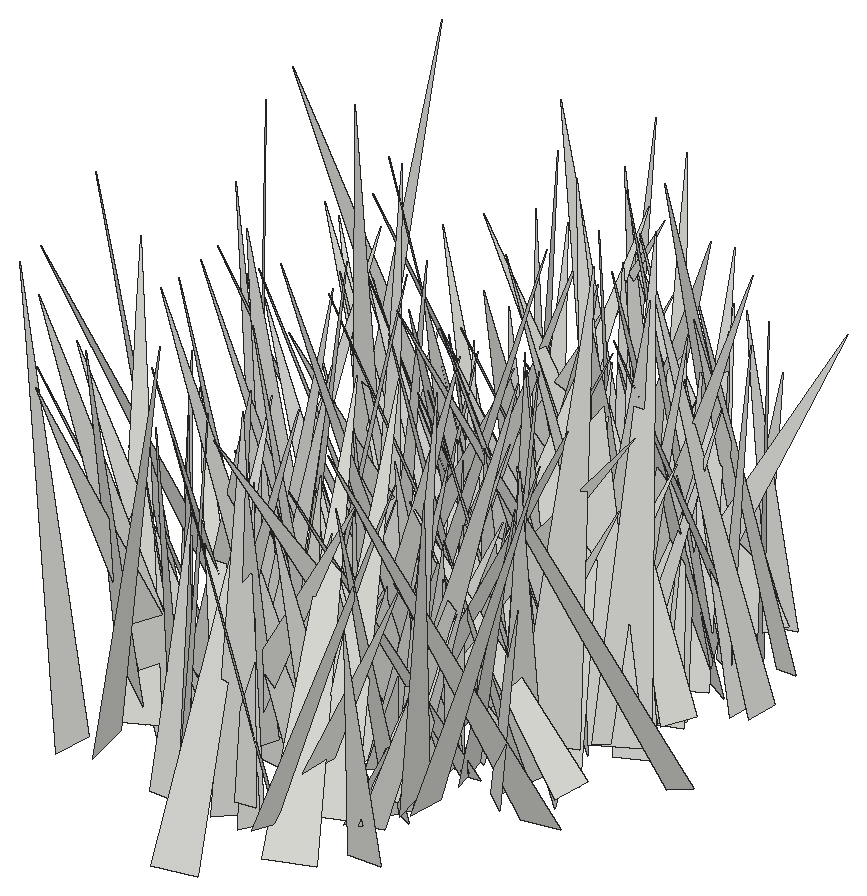
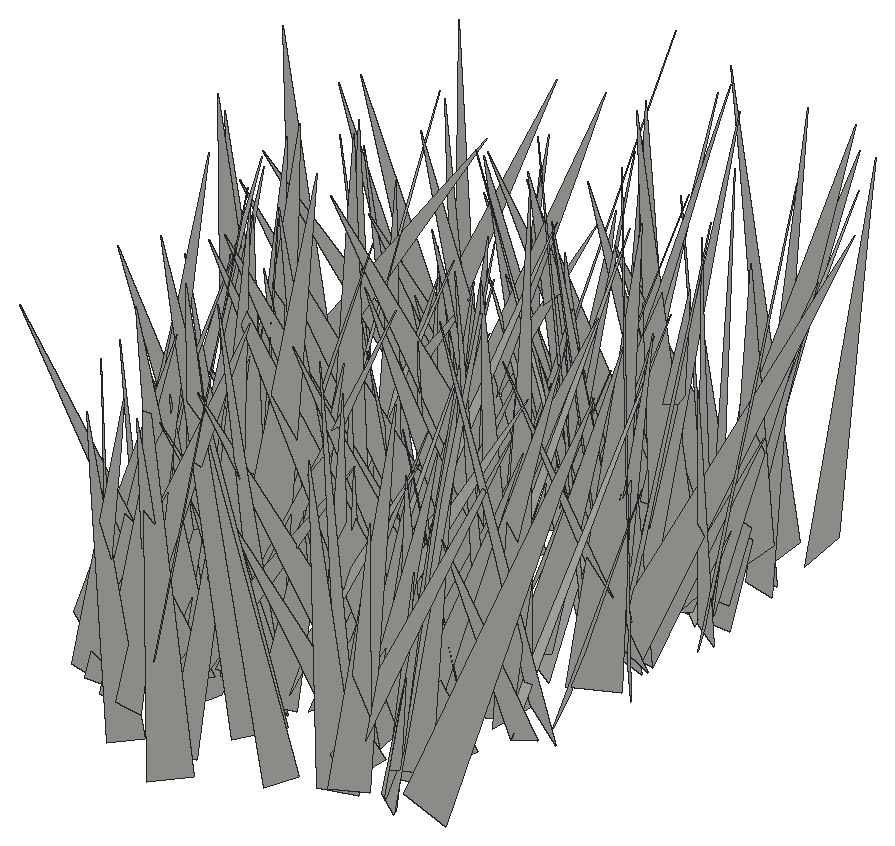
# SketchUp Ruby script. Lengths in inches.
U = 1.inch
M = Sketchup.active_model
def pt(a) = Geom::Point3d.new(a.map { |v| v * U })
def face(e, loops, mat)
  f = e.add_face(loops[0].map { |a| pt(a) })
  loops[1..].each { |l| e.add_face(l.map { |a| pt(a) }).erase! }
  f.material = f.back_material = mat if mat
  f
end
# faces: each face lists its corners as indices into pts; further lists are holes
def faces(e, pts, list, mat = nil) = list.each { |f| face(e, (f[0].is_a?(Array) ? f : [f]).map { |l| l.map { |i| pts[i] } }, mat) }
# xy, xz, yz: faces in a plane at the given z, y or x. An outline is a flat list of corners, or four numbers for a rectangle; further outlines are holes
def ring(l) = l.size == 4 ? [[l[0], l[1]], [l[2], l[1]], [l[2], l[3]], [l[0], l[3]]] : l.each_slice(2).to_a
def flat(e, list, mat, &to3) = list.each { |f| face(e, (f[0].is_a?(Array) ? f : [f]).map { |l| ring(l).map { |u, v| to3.(u, v) } }, mat) }
def xy(e, z, list, mat = nil) = flat(e, list, mat) { |x, y| [x, y, z] }
def xz(e, y, list, mat = nil) = flat(e, list, mat) { |x, z| [x, y, z] }
def yz(e, x, list, mat = nil) = flat(e, list, mat) { |y, z| [x, y, z] }
def lines(e, pts, list) = list.each { |a, b| e.add_line(pt(pts[a]), pt(pts[b])) }
# prism: a flat outline (further loops are holes) pulled along v
def prism(e, loops, v, mat = nil)
  f = face(e, loops, mat); d = Geom::Vector3d.new(v.map { |x| x * U })
  f.pushpull(f.normal.samedirection?(d) ? d.length : -d.length)
end
def box(e, o, s, mat = nil) = prism(e, [[o, [o[0] + s[0], o[1], o[2]], [o[0] + s[0], o[1] + s[1], o[2]], [o[0], o[1] + s[1], o[2]]]], [0, 0, s[2]], mat)
def at(x, y, z, deg = 0) = Geom::Transformation.translation(pt([x, y, z])) * Geom::Transformation.rotation(ORIGIN, Z_AXIS, deg.degrees)
def axes(o, x, y, z) = Geom::Transformation.new([*x, 0, *y, 0, *z, 0, *pt(o).to_a, 1])
def part(name) = M.definitions.add(name)
# library, detail: a bought-in or finely detailed component or shape, given as its bounding box
def library(name, o, s) = part(name).tap { |d| box(d.entities, o, s) }
def detail(e, o, s) = box(e.add_group.entities, o, s)
def put(e, d, t, mat = nil) = e.add_instance(d, t).tap { |i| i.material = mat if mat }
def group(e, t, mat = nil) = e.add_group.tap { |g| g.transformation = t; g.material = mat if mat }.entities
root = M.entities
c1 = part("fur_instance\#9")
p = [[0.8125,0,1.79],[0.67,-0.02,1.48],[0,-0.11,0],[0,0.11,0]]
faces(c1.entities,p,[[0,1,2,3]])
put(root,c1,axes([64.6,109.23,-27.1],[-0.79345,-6.87819,1.77521],[-6.83318,0.25089,-2.08208],[-1.94125,1.92821,6.60333]))
put(root,c1,axes([64.78,96.99,-27.1],[-6.58446,-3.61184,1.85584],[-3.84727,6.67992,-0.64953],[1.29924,1.4758,7.48189]))
put(root,c1,axes([66.12,98.6,-27.1],[-2.71774,-6.73125,0.47193],[-6.54696,2.5072,-1.9416],[-1.63394,1.15011,6.99472]))
put(root,c1,axes([65.09,91.46,-27.1],[-7.05246,-0.20222,1.59365],[-0.38202,7.18084,-0.77939],[1.56034,0.84409,7.01218]))
put(root,c1,axes([66.34,101.17,-28.22],[-5.41168,-1.42657,0.35166],[-1.45652,5.03228,-1.99993],[-0.1932,2.0214,5.22701]))
put(root,c1,axes([64.6875,96.98,-27.1],[1.72426,4.07776,1.35625],[4.04188,-2.03524,0.98061],[-1.4597,-0.81871,4.31736]))
put(root,c1,axes([65.79,93.5625,-27.1],[-1.06159,6.87885,0.56166],[6.76624,0.92524,1.45707],[-1.36093,-0.76575,6.80607]))
put(root,c1,axes([65.8,96.19,-27.1],[-4.26864,3.3889,1.68719],[3.78174,3.93314,1.66776],[0.17248,-2.36607,5.18889]))
put(root,c1,axes([66.37,104.19,-27.1],[-3.43494,4.07646,0.13435],[4.04677,3.38429,0.77755],[-0.50915,-0.60283,5.27368]))
put(root,c1,axes([64.64,100.35,-27.1],[-5.7343,-4.84539,3.53032],[-5.45543,6.24306,-0.29262],[2.4858,2.5238,7.50162]))
put(root,c1,axes([65.6,104.33,-27.1],[-4.61159,-4.4726,0.38091],[-4.39573,4.61032,0.9157],[0.90928,-0.396,6.35865]))
put(root,c1,axes([65.06,103.58,-27.1],[3.59561,7.30217,1.1805],[7.09033,-3.77639,1.76345],[-2.10771,-0.24675,7.94609]))
put(root,c1,axes([65.57,96.5,-27.1],[-4.43936,-4.76816,0.23664],[-4.66276,4.39992,1.18262],[1.02469,-0.63608,6.40661]))
put(root,c1,axes([66.47,97.26,-28.22],[-2.53868,-3.44184,0.53172],[-3.38696,2.28677,-1.36858],[-0.81085,1.22404,4.05193]))
put(root,c1,axes([67.52,105.47,-28.22],[-4.45593,-2.02584,0.38216],[-1.95722,3.87117,-2.29973],[-0.64758,2.23951,4.32095]))
put(root,c1,axes([67.875,97.15,-28.22],[-7.80069,-0.47128,0.71432],[-0.70737,7.23754,-2.94972],[0.48165,2.99651,7.23686]))
put(root,c1,axes([66.59,94.81,-28.22],[1.74253,-7.39949,2.19817],[-7.33714,-2.28781,-1.88496],[-2.39807,1.62304,7.36449]))
put(root,c1,axes([65.3,96.01,-27.1],[-2.6203,-2.567,1.06702],[-2.53846,2.80716,0.51965],[1.13325,0.35259,3.63117]))
put(root,c1,axes([65.17,101.21,-27.1],[3.62749,-5.55241,1.8821],[-5.65778,-3.89547,-0.58748],[-1.5366,1.23544,6.60627]))
put(root,c1,axes([64.91,104.55,-27.1],[-0.81178,3.59213,0.55552],[3.51446,0.92094,-0.81938],[0.92765,-0.34562,3.5904]))
put(root,c1,axes([66.1,95.3,-27.1],[2.22572,-6.24997,0.53761],[-6.03536,-2.28904,-1.62473],[-1.71046,-0.05581,6.43243]))
put(root,c1,axes([65.15,94.13,-27.1],[-2.48382,-6.27006,1.58629],[-6.2632,2.75568,1.08533],[1.61318,1.04494,6.65621]))
put(root,c1,axes([65.36,99.24,-27.1],[2.05142,5.93925,0.09208],[5.90467,-2.04959,0.65232],[-0.64654,0.12643,6.2496]))
put(root,c1,axes([66.57,98.1875,-27.1],[-5.55068,-3.03255,1.58004],[-3.06213,5.7489,0.27653],[1.52193,0.50669,6.31901]))
put(root,c1,axes([67.85,108.94,-27.1],[-3.27123,-4.88451,0.3113],[-4.82797,3.15879,-1.17003],[-0.80376,0.90546,5.76111]))
put(root,c1,axes([67.8,103.78,-27.1],[-5.5849,2.54638,0.93821],[2.66389,5.55377,0.78405],[0.51763,-1.10771,6.08773]))
put(root,c1,axes([65.93,103.79,-27.1],[7.3985,0.06507,3.2704],[0.28828,-8.06925,-0.49163],[-3.25831,-0.56619,7.38244]))
put(root,c1,axes([67.99,105.15,-27.1],[-4.93751,1.50851,0.32737],[1.53378,4.91815,0.47027],[0.1741,-0.54591,5.14135]))
put(root,c1,axes([67.68,100.77,-27.1],[-4.78062,2.36193,1.12593],[2.54726,4.73726,0.87783],[0.59826,-1.2963,5.25951]))
put(root,c1,axes([67.82,98.8,-28.22],[-3.1769,-1.92196,0.83625],[-2.09296,2.82701,-1.45378],[-0.11299,1.67333,3.4166]))
put(root,c1,axes([68.22,102.12,-28.22],[-4.63616,-0.58897,0.33378],[-0.62989,4.59941,-0.63319],[0.24806,0.67142,4.63033]))
put(root,c1,axes([66.77,108.02,-28.22],[-2.14945,-3.42966,1.0737],[-3.50191,2.27993,0.27214],[0.80747,0.75821,4.03839]))
put(root,c1,axes([68.64,102.91,-28.22],[-5.59376,-1.56322,0.76508],[-1.67452,5.53596,-0.93185],[0.47433,1.10847,5.73284]))
put(root,c1,axes([66.42,97.64,-28.22],[-0.60793,-4.00143,1.69165],[-4.28266,0.83877,0.44495],[0.72934,1.58988,4.02282]))
put(root,c1,axes([66.83,108.05,-28.22],[-4.90749,-6.3294,1.61985],[-6.13533,5.16095,1.5783],[2.24565,0.26836,7.85199]))
put(root,c1,axes([66.21,107.83,-27.1],[3.84252,-3.67557,0.42443],[-3.56655,-3.84235,-0.9854],[-0.98471,-0.42605,5.2253]))
put(root,c1,axes([65.84,92.09,-27.1],[6.8953,0.9557,1.85973],[1.13553,-7.09282,-0.56526],[-1.75571,-0.83402,6.93822]))
put(root,c1,axes([66.9375,94.19,-28.22],[-4.85936,-1.80324,2.4582],[-1.94231,5.39639,0.11902],[2.34986,0.73149,5.18178]))
put(root,c1,axes([67.98,106.21,-28.22],[1.10778,3.32388,1.25845],[3.28018,-1.46364,0.97838],[-1.36832,-0.8177,3.36424]))
put(root,c1,axes([67.26,108.86,-27.1],[1.04159,-3.44564,1.2731],[-3.64709,-1.12789,-0.06873],[-0.4381,1.19732,3.59897]))
put(root,c1,axes([67.01,97.08,-27.1],[-3.15588,-6.30761,0.73503],[-6.08642,3.23856,1.65924],[1.81157,-0.10755,6.85511]))
put(root,c1,axes([66.91,93.83,-27.1],[4.97052,1.68586,2.30908],[2.28367,-5.12743,-1.17229],[-1.72012,-1.9358,5.11604]))
put(root,c1,axes([68.53,102.11,-27.1],[-4.85913,-4.7221,0.69622],[-4.68141,4.90862,0.61965],[0.93132,0.03646,6.74725]))
put(root,c1,axes([69.16,105.54,-27.1],[-5.26641,1.25593,0.32091],[1.22212,5.2582,-0.5227],[0.43216,0.43524,5.3888]))
put(root,c1,axes([66.55,98,-28.22],[2.76981,6.05425,2.08045],[6.39697,-2.70498,-0.64491],[-0.24704,-2.16406,6.62646]))
put(root,c1,axes([67.95,99.92,-28.22],[-3.01664,-4.03882,0.35129],[-3.9528,3.02747,0.86334],[0.90049,-0.2406,4.96657]))
put(root,c1,axes([69.95,97.88,-27.1],[-6.57116,-2.81105,0.67584],[-2.85659,6.57143,-0.44162],[0.44572,0.67315,7.13352]))
put(root,c1,axes([68.75,100.75,-27.1],[1.63726,6.8228,1.57078],[6.72877,-1.9791,1.58281],[-1.9343,-1.10957,6.83563]))
put(root,c1,axes([67.66,92.32,-28.22],[0.08928,4.21713,1.27448],[4.4055,-0.088,-0.01741],[-0.00879,-1.27457,4.21804]))
put(root,c1,axes([66.88,109.67,-27.1],[4.17409,-3.35782,0.27535],[-3.2273,-4.11088,-1.20788],[-0.96712,-0.77425,5.2191]))
put(root,c1,axes([69.53,93.34,-28.22],[-2.82943,5.24506,0.49337],[5.22615,2.72388,1.01368],[-0.66438,-0.91081,5.87271]))
put(root,c1,axes([69.28,104.125,-28.22],[0.6668,-6.36542,0.43774],[-6.10772,-0.7641,-1.80742],[-1.84553,0.22889,6.13974]))
put(root,c1,axes([66.49,99.875,-27.1],[5.45903,4.38742,2.52703],[5.0114,-5.21201,-1.77686],[-0.72192,-3.00365,6.77446]))
put(root,c1,axes([67.1,103.46,-27.1],[3.49606,4.56093,2.47636],[5.16488,-3.35013,-1.12142],[-0.50841,-2.67048,5.63622]))
put(root,c1,axes([67.91,92.8125,-28.22],[3.99026,4.07334,2.14881],[4.32029,-4.29562,0.12027],[-1.59518,-1.44473,5.70086]))
put(root,c1,axes([66.04,96.46,-27.1],[2.61473,-6.42495,0.46001],[-6.33227,-2.47287,1.45453],[1.18065,0.96609,6.78241]))
put(root,c1,axes([67.32,103.91,-28.22],[3.51843,3.11531,1.14482],[3.25687,-3.56198,-0.31656],[-0.63919,-1.00114,4.68874]))
put(root,c1,axes([68.3,108.38,-28.22],[-1.35199,5.16754,1.66066],[5.39955,1.4549,-0.13134],[0.55327,-1.57128,5.33986]))
put(root,c1,axes([71.45,103.36,-27.1],[-4.82792,-3.85999,0.34861],[-3.62589,4.30173,-2.58417],[-1.36894,2.21934,5.6152]))
put(root,c1,axes([67.25,106.76,-28.22],[-1.80775,-6.68688,0.47497],[-6.40102,1.86794,1.93536],[1.9917,-0.06601,6.65106]))
put(root,c1,axes([68.8,104.51,-28.22],[-1.17354,4.22506,1.16991],[4.38332,1.15287,0.2334],[0.0799,-1.19029,4.3788]))
put(root,c1,axes([67.4375,97.3125,-27.1],[1.6675,5.06938,1.93589],[5.41393,-1.41673,-0.95346],[0.36831,-2.12629,5.25072]))
put(root,c1,axes([68.26,107.84,-28.22],[-0.44013,-4.40012,0.04518],[-4.35564,0.44209,0.62427],[0.62566,-0.01764,4.37779]))
put(root,c1,axes([70.5,95.12,-27.1],[-7.46338,-1.41905,1.28497],[-1.31215,7.55774,0.72509],[1.39396,-0.48353,7.56241]))
put(root,c1,axes([69.37,106.61,-28.22],[-6.13991,-1.94187,2.86824],[-2.65031,6.39227,-1.34568],[2.23013,2.25037,6.2975]))
put(root,c1,axes([68.12,93,-28.22],[6.19902,-0.22924,1.58295],[-0.50577,-6.29178,1.06951],[-1.51739,1.16065,6.11037]))
put(root,c1,axes([70.38,106.66,-27.1],[-4.26767,-0.91045,0.71231],[-0.70932,4.21373,1.13607],[0.91278,-0.98229,4.21323]))
put(root,c1,axes([70.15,101.77,-28.22],[-2.65941,2.49787,0.36396],[2.46932,2.68404,-0.37765],[0.52369,0.0288,3.62894]))
put(root,c1,axes([70.5625,89.17,-28.22],[-5.84983,3.65343,0.11485],[3.32744,5.4123,-2.68634],[1.51292,2.22277,6.35229]))
put(root,c1,axes([71.56,106.9,-27.1],[-3.04212,-3.44962,0.11938],[-3.35963,2.92271,-1.15727],[-0.79185,0.85236,4.45141]))
put(root,c1,axes([68.73,96.44,-28.22],[2.18192,-3.03993,1.35648],[-3.32882,-1.9865,0.90262],[0.01238,1.6293,3.63142]))
put(root,c1,axes([71.01,95.46,-27.1],[-6.09908,-2.25868,1.59557],[-2.41433,6.23322,-0.4051],[1.3485,0.94419,6.49124]))
put(root,c1,axes([71.0625,98.69,-28.22],[-0.15517,3.72025,1.9318],[3.94772,-0.52047,1.31942],[-1.40985,-1.86683,3.48188]))
put(root,c1,axes([68.74,102.37,-28.22],[6.5419,0.41912,1.71437],[-0.23349,-6.31856,2.43568],[-1.74935,2.41069,6.08602]))
put(root,c1,axes([70.61,92.44,-28.22],[-3.88558,0.60859,0.85055],[0.43871,3.91906,-0.80001],[0.9494,0.67978,3.85072]))
put(root,c1,axes([70.99,91.83,-27.1],[0.97276,4.45119,0.9772],[4.35496,-1.20232,1.14148],[-1.3425,-0.67498,4.41093]))
put(root,c1,axes([71.98,103.91,-28.22],[-6.71472,0.14595,1.05093],[-0.21339,6.41005,-2.25365],[1.03933,2.25902,6.32691]))
put(root,c1,axes([71.66,96.22,-28.22],[-3.92921,-1.09616,0.24918],[-1.11465,3.91653,-0.34741],[0.14562,0.40197,4.06442]))
put(root,c1,axes([67.83,101.59,-27.1],[5.28703,-2.12696,0.17156],[-2.11759,-5.17319,1.12251],[0.26309,1.10465,5.58719]))
put(root,c1,axes([69.21,94.63,-27.1],[4.90376,-2.85552,0.72078],[-2.73926,-4.93651,-0.92072],[-1.08166,-0.44414,5.59939]))
put(root,c1,axes([69.9375,92.79,-28.22],[-4.38219,4.14776,3.28171],[4.71988,4.98997,-0.0042],[2.38668,-2.25242,6.03386]))
put(root,c1,axes([69.72,95.63,-27.1],[2.82184,-3.33686,1.43593],[-3.57868,-2.86589,0.37288],[-0.62414,1.34588,4.35412]))
put(root,c1,axes([69.68,95.5,-28.22],[5.71474,5.0925,1.62445],[5.00095,-5.93344,1.00766],[-1.88756,-0.30227,7.58791]))
put(root,c1,axes([72.32,102.2,-28.22],[-5.16383,-5.19186,0.43743],[-5.2089,5.15828,-0.26709],[0.11856,0.49863,7.31773]))
put(root,c1,axes([70.96,93.27,-28.22],[-4.71687,-4.84842,1.35584],[-4.8132,4.8877,0.73342],[1.47602,0.44449,6.72444]))
put(root,c1,axes([71.3125,103.89,-28.22],[-4.54245,-0.30979,1.16713],[-0.64985,4.4561,-1.34644],[1.01777,1.46262,4.34936]))
put(root,c1,axes([71.08,104.77,-28.22],[-3.58338,-3.97137,0.418],[-3.89573,3.60001,0.80641],[0.87736,-0.23507,5.28792]))
put(root,c1,axes([71.45,101.7,-27.1],[-3.14093,-4.54056,1.19879],[-4.68857,3.11384,-0.49041],[0.26658,1.26749,5.49924]))
put(root,c1,axes([68.88,95.65,-28.22],[1.41484,-4.55258,1.06253],[-4.54528,-1.07998,1.42506],[1.09333,1.40157,4.54939]))
put(root,c1,axes([66.92,105.38,-28.22],[6.5519,-4.81181,0.9912],[-4.80718,-5.93833,2.94799],[1.01342,2.94042,7.57563]))
put(root,c1,axes([68.43,106.79,-28.22],[3.29977,-2.51906,0.3221],[-2.3698,-2.86445,1.87534],[0.91296,1.66948,3.70368]))
put(root,c1,axes([70.18,105.66,-27.1],[3.44775,-2.42349,1.09947],[-2.43313,-3.5995,-0.30427],[-1.07797,0.37336,4.2033]))
put(root,c1,axes([67.88,94.18,-28.22],[4.35594,-4.3452,0.48537],[-4.22774,-4.01128,2.03138],[1.11472,1.7662,5.80763]))
put(root,c1,axes([70.33,98.45,-28.22],[-1.39495,-5.41554,1.57218],[-5.52882,1.63221,0.71678],[1.10996,1.3242,5.54619]))
put(root,c1,axes([69.03,105.06,-28.22],[6.04009,-0.71684,0.90558],[-1.00409,-5.64184,2.23115],[-0.57074,2.3393,5.65849]))
put(root,c1,axes([69.32,96.4,-28.22],[4.85217,1.44436,0.49792],[1.4914,-4.83766,-0.50049],[-0.33141,-0.62336,5.03778]))
put(root,c1,axes([72.125,96.05,-27.1],[-3.54918,2.04608,0.76374],[2.14815,3.53344,0.51649],[0.39398,-0.83357,4.06404]))
put(root,c1,axes([71.25,107.3,-27.1],[1.69834,-4.62751,0.65795],[-4.61755,-1.76962,-0.52709],[-0.72459,0.43091,4.90106]))
put(root,c1,axes([70.83,99.14,-27.1],[-6.33754,-5.19611,0.8236],[-4.02771,5.62162,4.47406],[3.3846,-3.03975,6.86635]))
put(root,c1,axes([71.38,94.96,-27.1],[3.60801,-2.69307,1.35493],[-2.4926,-3.85347,-1.02171],[-1.69571,-0.06573,4.3848]))
put(root,c1,axes([74.25,106.78,-28.22],[-7.38136,0.22251,0.33251],[0.26326,7.32737,0.9407],[0.30128,-0.95116,7.32455]))
put(root,c1,axes([69.84,108.89,-28.22],[4.67852,-1.7119,0.20248],[-1.71617,-4.68064,0.08066],[-0.16239,0.14538,4.98123]))
put(root,c1,axes([74.28,97.09,-27.1],[1.30343,6.50873,4.51627],[7.0846,-3.00591,2.28737],[-3.54523,-3.61388,6.23141]))
put(root,c1,axes([69.01,106.84,-28.22],[7.07591,-3.11018,0.05148],[-3.09924,-7.06002,-0.5432],[-0.26559,-0.47663,7.71016]))
put(root,c1,axes([74.09,107.92,-27.1],[-1.49578,-4.28811,0.26565],[-3.87905,1.22698,-2.03551],[-1.84701,0.89578,4.0598]))
put(root,c1,axes([72.86,106.625,-27.1],[1.59006,-7.38899,3.46765],[-7.94346,-2.21328,-1.07372],[-1.87702,3.10714,7.48148]))
put(root,c1,axes([73.46,98.82,-28.22],[-2.18116,-3.44946,0.52539],[-3.41914,1.9894,-1.13316],[-0.6959,1.0372,3.92074]))
put(root,c1,axes([73.02,105.3,-28.22],[2.8075,7.47142,1.47372],[7.21104,-3.11318,2.04573],[-2.44844,-0.60171,7.71486]))
put(root,c1,axes([71.54,99.42,-27.1],[3.51488,-3.51732,0.75482],[-3.443,-3.59499,-0.71937],[-1.04262,0.01399,4.9202]))
put(root,c1,axes([72.79,91.5625,-28.22],[-3.48559,6.14429,0.41822],[6.11379,3.5101,-0.61419],[0.74073,-0.05879,7.03735]))
put(root,c1,axes([72.18,93.31,-27.1],[-2.71251,3.20119,0.88639],[3.03008,2.85354,-1.03292],[1.36084,0.02704,4.06674]))
put(root,c1,axes([70.97,96.95,-27.1],[6.40804,-1.16691,1.44574],[-1.35043,-6.49108,0.74636],[-1.27601,1.00946,6.47052]))
put(root,c1,axes([72.63,95.72,-27.1],[-6.96158,0.42843,3.50828],[-1.43896,6.73486,-3.67782],[3.22816,3.92599,5.92628]))
put(root,c1,axes([72.08,100.43,-27.1],[-4.61251,5.93847,1.25396],[5.3205,4.71401,-2.75381],[2.92064,0.79104,6.99694]))
put(root,c1,axes([73.32,92.69,-27.1],[-3.56616,5.34471,0.77163],[5.27091,3.64619,-0.89538],[1.17426,-0.13507,6.36253]))
put(root,c1,axes([74.94,96.95,-27.1],[-1.76635,-5.02439,0.02248],[-4.81779,1.68692,-1.51928],[-1.42615,0.52421,5.10454]))
put(root,c1,axes([72.37,96.12,-27.1],[4.7492,-0.22527,1.39473],[-0.44396,-4.88167,0.72329],[-1.34124,0.81823,4.6992]))
put(root,c1,axes([74.06,97.5,-27.1],[1.76698,3.75792,1.11012],[3.4505,-2.06932,1.51278],[-1.85698,-0.26926,3.86726]))
put(root,c1,axes([70.71,108.72,-27.1],[5.42547,-4.53511,0.52895],[-4.56014,-5.3411,0.98008],[0.2284,1.09004,7.00303]))
put(root,c1,axes([73.38,99.37,-28.22],[2.88186,3.44939,0.31018],[3.15851,-2.7832,1.60537],[-1.42067,0.8094,4.19835]))
put(root,c1,axes([72.2,91.125,-27.1],[5.46763,0.70402,1.09334],[0.38726,-5.3924,1.5356],[-1.2414,1.41859,5.29457]))
put(root,c1,axes([73.86,106.59,-27.1],[-6.94561,0.7265,2.56424],[0.79665,7.39636,0.06233],[2.54332,-0.33278,6.98322]))
put(root,c1,axes([72.92,99.3125,-27.1],[3.22488,1.438,0.95498],[1.40641,-3.36208,0.31327],[-1.00092,-0.09099,3.51704]))
put(root,c1,axes([75.65,103.56,-28.22],[-6.93543,-2.32629,0.88421],[-2.41004,6.93097,-0.66862],[0.62063,0.91853,7.28456]))
put(root,c1,axes([72.46,104.87,-27.1],[4.05537,2.07279,0.17475],[1.9711,-3.95155,1.12829],[-0.66463,0.92835,4.41242]))
put(root,c1,axes([73.28,95.73,-28.22],[-1.87294,-5.65903,1.00828],[-5.62978,2.02003,0.87988],[1.16052,0.66634,5.89562]))
put(root,c1,axes([72.13,97.34,-27.1],[0.15011,3.96157,1.30257],[3.86973,0.35348,-1.52101],[1.55431,-1.26265,3.66102]))
put(root,c1,axes([72.41,98.08,-28.22],[2.83156,-3.99697,0.33188],[-4.00855,-2.80696,0.39506],[0.13188,0.49882,4.88236]))
put(root,c1,axes([71.71,92.85,-28.22],[4.56637,-2.19972,0.30987],[-2.21681,-4.46657,0.96025],[0.14341,0.99877,4.97679]))
put(root,c1,axes([72.83,109.4375,-28.22],[-1.84691,-6.18778,0.26193],[-5.9057,1.84189,1.87043],[1.86547,-0.29517,6.18071]))
put(root,c1,axes([74.34,104.44,-27.1],[-5.53367,-3.1899,2.46645],[-3.58117,5.81278,-0.51687],[1.85312,1.70777,6.3663]))
put(root,c1,axes([74.79,99.58,-28.22],[-3.99864,-1.03805,0.42764],[-0.78188,3.71014,1.695],[0.80565,-1.55139,3.76744]))
put(root,c1,axes([72.28,110.65,-28.22],[4.90607,-3.46037,0.24315],[-3.44997,-4.91123,-0.28332],[-0.36191,-0.09172,5.99695]))
put(root,c1,axes([76.48,98.87,-28.22],[-5.23852,-3.39609,0.6769],[-3.443,4.97658,-1.67721],[-0.37061,1.77027,6.01352]))
put(root,c1,axes([76.1875,108.58,-27.1],[-3.70212,4.89762,1.86065],[5.19102,3.12087,2.11373],[-0.70854,-2.72541,5.76407]))
put(root,c1,axes([72.9,100.67,-28.22],[5.82388,-2.11588,0.96568],[-1.89422,-5.82584,-1.34106],[-1.34958,-0.95373,6.04946]))
put(root,c1,axes([72.59,102.62,-28.22],[2.24537,-6.9608,0.71668],[-6.96969,-2.1575,0.8813],[0.62434,0.94895,7.26069]))
put(root,c1,axes([73.64,95.86,-27.1],[-2.04646,-5.42862,2.85461],[-5.95901,2.47232,0.42963],[1.45222,2.49488,5.78561]))
put(root,c1,axes([74.72,102.52,-28.22],[-6.10663,-5.12788,1.30944],[-4.81653,6.21333,1.86984],[2.19336,-0.63253,7.75176]))
put(root,c1,axes([76,104.15,-28.22],[0.27633,8.1596,0.76138],[7.93766,-0.45592,2.00518],[-2.0377,-0.66947,7.91421]))
put(root,c1,axes([70.28,99.93,-27.1],[4.62991,-4.98565,0.093],[-4.3743,-3.99984,3.34189],[2.39393,2.33366,5.92659]))
put(root,c1,axes([74.33,104.91,-28.22],[-4.98307,4.13485,3.06586],[4.6284,5.46651,0.15019],[2.25263,-2.08511,6.47344]))
put(root,c1,axes([72.86,106.48,-27.1],[5.93446,-4.51627,0.11992],[-4.41947,-5.84426,-1.3935],[-0.93776,-1.03771,7.32616]))
put(root,c1,axes([73.6875,94.64,-27.1],[-0.65991,4.20046,0.70673],[4.09857,0.8209,-1.05196],[1.15975,-0.51096,4.1198]))
put(root,c1,axes([74.25,97.1,-27.1],[-3.40135,-0.48301,1.73948],[-0.24917,3.80046,0.56808],[1.78802,-0.38922,3.38818]))
put(root,c1,axes([75.13,107.43,-27.1],[-0.50295,4.78104,0.71911],[4.81704,0.43358,0.48636],[-0.41423,-0.76294,4.78276]))
put(root,c1,axes([75.875,106.6875,-27.1],[-6.16765,-3.82155,1.90605],[-3.98751,6.35208,-0.16723],[1.52874,1.15063,7.2537]))
put(root,c1,axes([74.77,101.29,-27.1],[2.46831,-3.73303,1.12427],[-3.72872,-2.64901,-0.60947],[-1.13849,0.58247,4.43358]))
put(root,c1,axes([74.67,109.81,-27.1],[-1.5232,-7.73744,1.34983],[-7.81047,1.63722,0.57115],[0.82858,1.20901,7.86523]))
put(root,c1,axes([74.58,93.01,-27.1],[5.42,0.95377,1.93695],[-0.10115,-5.11614,2.80228],[-2.15667,2.63692,4.73638]))
put(root,c1,axes([72.9,94.51,-28.22],[7.74445,1.42991,0.81828],[1.0012,-7.20795,3.11989],[-1.30836,2.94814,7.231]))
put(root,c1,axes([73.28,95.4,-28.22],[7.18053,-1.42617,1.70446],[-1.71997,-7.21687,1.20732],[-1.40743,1.54336,7.22055]))
put(root,c1,axes([74.33,92.97,-28.22],[0.91835,-4.65892,0.5996],[-4.68613,-0.86646,0.44487],[0.32448,0.67241,4.72768]))
put(root,c1,axes([75.24,106.09,-28.22],[-4.06355,5.05875,1.67662],[5.05755,4.32523,-0.79246],[1.68023,-0.78477,6.44014]))
put(root,c1,axes([77.625,98.11,-27.1],[-3.75948,2.94392,0.27379],[2.73653,3.29698,2.12525],[-1.1194,-1.82718,4.27594]))
put(root,c1,axes([77.01,100.87,-27.1],[-1.50956,7.97784,1.83345],[8.07703,1.14872,1.65178],[-1.3301,-2.07864,7.94961]))
put(root,c1,axes([76.15,98.2,-28.22],[-1.9055,-4.08481,0.78377],[-4.15591,1.83492,-0.5407],[-0.16841,0.93717,4.47485]))
put(root,c1,axes([73.58,104.69,-28.22],[6.69974,-1.69034,1.74311],[-2.11177,-6.58131,1.73465],[-1.19837,2.1474,6.68841]))
put(root,c1,axes([74.2,104.86,-27.1],[-1.49797,-4.88201,2.75569],[-5.27998,2.18724,1.00478],[1.88406,2.24805,5.00683]))
put(root,c1,axes([76.91,97.65,-28.22],[-0.88458,-7.33954,0.10795],[-7.20369,0.84713,-1.43254],[-1.40973,0.27658,7.25253]))
put(root,c1,axes([75.73,99.88,-28.22],[-1.14776,6.0133,0.84328],[6.0716,1.14805,0.07727],[0.08148,-0.84289,6.12137]))
put(root,c1,axes([75.59,106.91,-28.22],[-3.21608,-6.87634,1.40534],[-6.91778,3.36666,0.64196],[1.18463,0.99184,7.56406]))
put(root,c1,axes([76.16,104.47,-28.22],[-5.1152,1.11044,1.16629],[0.73583,5.06638,-1.59654],[1.43244,1.36283,4.98492]))
put(root,c1,axes([73.76,99.5,-27.1],[3.57113,-2.0967,0.79041],[-2.23153,-3.1932,1.61171],[0.20288,1.78359,3.81464]))
put(root,c1,axes([74.54,109.74,-28.22],[2.7967,-3.72992,1.22325],[-3.91864,-2.74089,0.60164],[-0.23004,1.34365,4.62297]))
put(root,c1,axes([76.47,109.04,-27.1],[-0.19493,4.51759,1.73565],[4.75586,-0.14282,0.90585],[-0.89608,-1.74071,4.43013]))
put(root,c1,axes([75.68,109.23,-27.1],[0.67121,-5.58126,0.90748],[-5.6399,-0.72653,-0.2969],[-0.40679,0.86382,5.61363]))
put(root,c1,axes([74.47,101.48,-27.1],[0.4921,4.23207,0.57816],[4.10963,-0.31046,-1.22532],[1.16432,-0.69285,4.08059]))
put(root,c1,axes([79.92,100.11,-27.1],[-3.41379,-7.32141,0.63154],[-6.65452,2.7845,-3.69049],[-3.11756,2.07349,7.18591]))
put(root,c1,axes([75.2,103.33,-28.22],[1.79121,4.66243,0.42191],[4.67903,-1.79759,0.00003],[-0.15134,-0.39383,4.99466]))
put(root,c1,axes([74.33,103.4,-28.22],[5.72788,-5.11466,1.67521],[-5.30647,-5.77538,0.51083],[-0.89854,1.50329,7.66207]))
put(root,c1,axes([76.65,102.22,-28.22],[1.5886,-5.12639,3.23902],[-5.9044,-2.07062,-0.3813],[-1.38174,2.95423,5.35333]))
put(root,c1,axes([76.36,96.29,-27.1],[3.82909,4.88275,1.88302],[4.81565,-4.20088,1.10051],[-2.04855,-0.74856,6.10673]))
put(root,c1,axes([76.1,108.47,-28.22],[4.38059,2.58911,2.20412],[2.75267,-4.81057,0.18002],[-1.99611,-0.9519,5.08534]))
put(root,c1,axes([74.5625,94.94,-27.1],[6.47505,-0.26988,1.20187],[0.07267,-6.33614,-1.81428],[-1.22965,-1.79557,6.22153]))
put(root,c1,axes([77.26,106.23,-28.22],[-4.97388,0.03891,0.99351],[0.0174,5.07103,-0.11152],[0.99411,0.10595,4.97278]))
put(root,c1,axes([74.8125,97.0625,-27.1],[5.2345,0.58731,0.96902],[0.7581,-5.21929,-0.93179],[-0.84215,-1.04786,5.18428]))
put(root,c1,axes([78.98,104.93,-27.1],[-7.05105,-1.29004,0.36767],[-1.33665,6.92247,-1.34515],[0.11284,1.38992,7.04075]))
put(root,c1,axes([78.07,107.16,-27.1],[-2.85535,-4.62994,1.75531],[-4.89429,2.33192,-1.81068],[-0.75056,2.40755,5.12941]))
put(root,c1,axes([75.49,99.75,-27.1],[-3.47226,6.33449,3.63746],[6.89094,4.17667,-0.69553],[2.42317,-2.80055,7.19017]))
put(root,c1,axes([77.51,103.07,-27.1],[-4.02277,2.62654,1.01722],[2.78428,3.97624,0.74391],[0.42575,-1.18612,4.74637]))
put(root,c1,axes([75.1,99.03,-28.22],[5.78336,-2.78291,1.02515],[-2.6557,-5.85961,-0.92463],[-1.32013,-0.40388,6.35113]))
put(root,c1,axes([73.89,107.32,-27.1],[1.55014,5.60518,1.20615],[5.3228,-0.94254,-2.46072],[2.13086,-1.72318,5.26933]))
put(root,c1,axes([76.34,107.47,-27.1],[-2.99336,-6.46525,0.18966],[-6.30073,2.9619,1.52434],[1.46161,-0.47255,6.9596]))
put(root,c1,axes([76.5,106.34,-27.1],[2.39277,4.07076,1.54907],[4.21231,-2.6123,0.35825],[-1.10775,-1.14055,4.7083]))
put(root,c1,axes([75.03,94.84,-27.1],[6.15775,0.09619,0.89999],[0.03195,-6.20791,0.44493],[-0.90455,0.43558,6.14241]))
put(root,c1,axes([77.02,101.13,-27.1],[-5.99811,4.4385,2.51735],[4.45899,6.44808,-0.74453],[2.48087,-0.8583,7.4245]))
